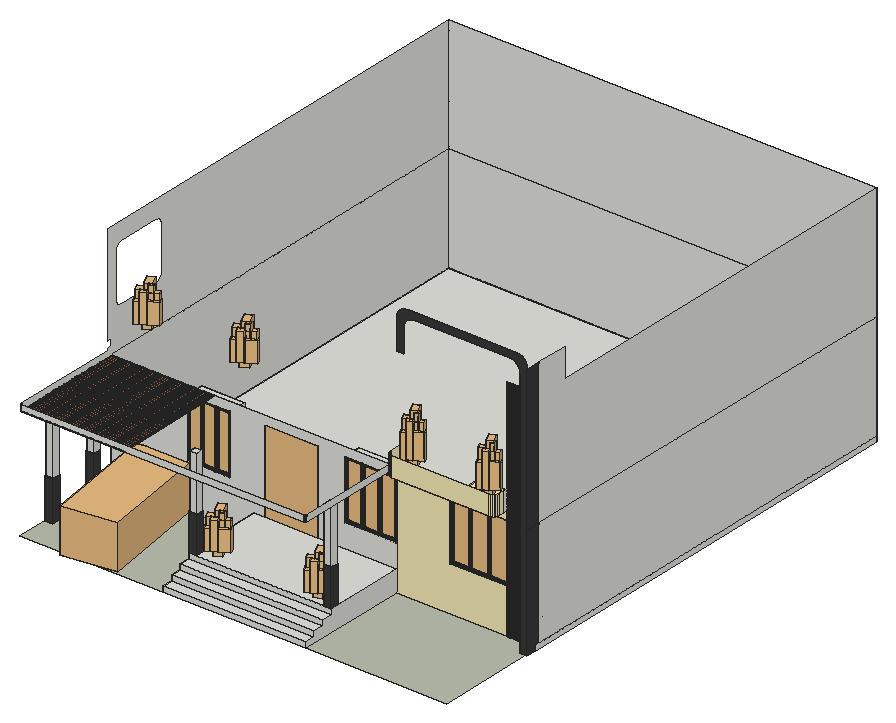
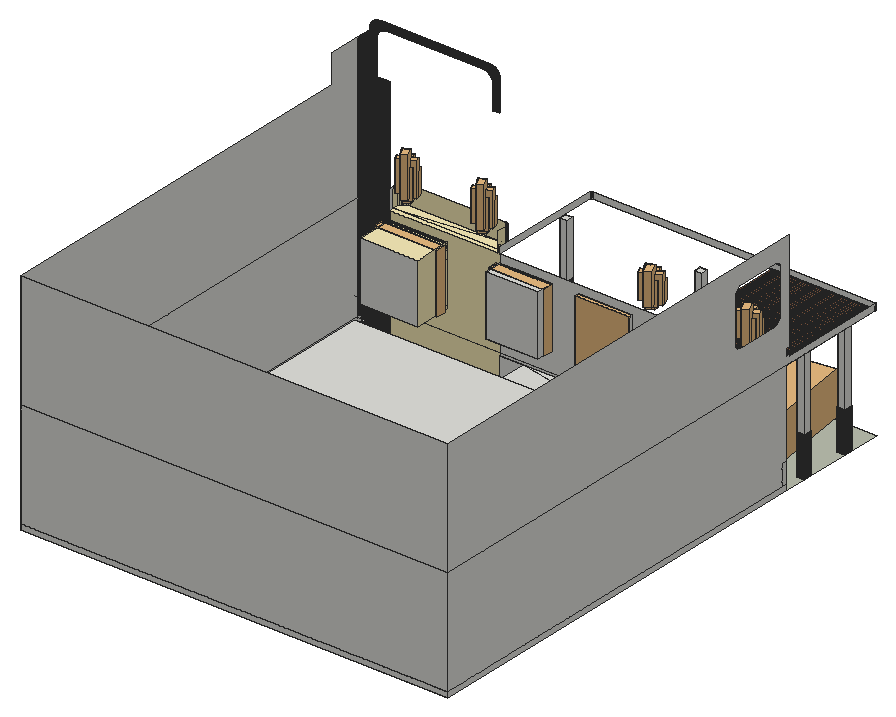
# SketchUp Ruby script. Lengths in inches.
U = 1.inch
M = Sketchup.active_model
def pt(a) = Geom::Point3d.new(a.map { |v| v * U })
def face(e, loops, mat)
  f = e.add_face(loops[0].map { |a| pt(a) })
  loops[1..].each { |l| e.add_face(l.map { |a| pt(a) }).erase! }
  f.material = f.back_material = mat if mat
  f
end
# faces: each face lists its corners as indices into pts; further lists are holes
def faces(e, pts, list, mat = nil) = list.each { |f| face(e, (f[0].is_a?(Array) ? f : [f]).map { |l| l.map { |i| pts[i] } }, mat) }
# xy, xz, yz: faces in a plane at the given z, y or x. An outline is a flat list of corners, or four numbers for a rectangle; further outlines are holes
def ring(l) = l.size == 4 ? [[l[0], l[1]], [l[2], l[1]], [l[2], l[3]], [l[0], l[3]]] : l.each_slice(2).to_a
def flat(e, list, mat, &to3) = list.each { |f| face(e, (f[0].is_a?(Array) ? f : [f]).map { |l| ring(l).map { |u, v| to3.(u, v) } }, mat) }
def xy(e, z, list, mat = nil) = flat(e, list, mat) { |x, y| [x, y, z] }
def xz(e, y, list, mat = nil) = flat(e, list, mat) { |x, z| [x, y, z] }
def yz(e, x, list, mat = nil) = flat(e, list, mat) { |y, z| [x, y, z] }
def lines(e, pts, list) = list.each { |a, b| e.add_line(pt(pts[a]), pt(pts[b])) }
# prism: a flat outline (further loops are holes) pulled along v
def prism(e, loops, v, mat = nil)
  f = face(e, loops, mat); d = Geom::Vector3d.new(v.map { |x| x * U })
  f.pushpull(f.normal.samedirection?(d) ? d.length : -d.length)
end
def box(e, o, s, mat = nil) = prism(e, [[o, [o[0] + s[0], o[1], o[2]], [o[0] + s[0], o[1] + s[1], o[2]], [o[0], o[1] + s[1], o[2]]]], [0, 0, s[2]], mat)
def at(x, y, z, deg = 0) = Geom::Transformation.translation(pt([x, y, z])) * Geom::Transformation.rotation(ORIGIN, Z_AXIS, deg.degrees)
def axes(o, x, y, z) = Geom::Transformation.new([*x, 0, *y, 0, *z, 0, *pt(o).to_a, 1])
def part(name) = M.definitions.add(name)
# library, detail: a bought-in or finely detailed component or shape, given as its bounding box
def library(name, o, s) = part(name).tap { |d| box(d.entities, o, s) }
def detail(e, o, s) = box(e.add_group.entities, o, s)
def put(e, d, t, mat = nil) = e.add_instance(d, t).tap { |i| i.material = mat if mat }
def group(e, t, mat = nil) = e.add_group.tap { |g| g.transformation = t; g.material = mat if mat }.entities
root = M.entities
M.materials.add("0899 AP 7833 SUNKISSED").color = [249, 236, 185]
M.materials.add("POT_TEXTURE_1").color = [172, 172, 172]
M.materials.add("Wine2").color = [0, 0, 0]
M.materials["Wine2"].alpha = 0
M.materials.add("[0130_Gainsboro]").color = [39, 45, 50]
M.materials.add("[Color M07]").color = [58, 58, 58]
M.materials.add("[Pavers with Grass Brick]").color = [187, 192, 176]
M.materials.add("[Wood Veneer 02]").color = [190, 128, 91]
M.materials.add("soil1").color = [68, 55, 47]
c1 = part("Group381\#1")
prism(c1.entities,[[[-13,124.5,0],[-13,-124.5,0],[-14,-124.5,0],[-14,-80.5625,0],[-14,-13.875,0],[-14,-4.5,0],[-14,19.5,0],[-14,43.5,0],[-14,106.48,0],[-14,107.5,0],[-14,122.5625,0],[-14,124.5,0]]],[0,0,0.25])
c2 = part("Group382\#1")
box(c2.entities,[-12.6875,-124.5,0],[1,249,0.25])
c3 = part("Group383\#1")
box(c3.entities,[-11.375,-124.5,0],[1,249,0.25])
c4 = part("Group384\#1")
box(c4.entities,[-10.0625,-124.5,0],[1,249,0.25])
c5 = part("Group385\#1")
box(c5.entities,[-8.75,-124.5,0],[1,249,0.25])
c6 = part("Group386\#1")
box(c6.entities,[-7.4375,-124.5,0],[1,249,0.25])
c7 = part("Group387\#1")
box(c7.entities,[-6.125,-124.5,0],[1,249,0.25])
c8 = part("Group388\#1")
box(c8.entities,[-4.8125,-124.5,0],[1,249,0.25])
c9 = part("Group389\#1")
box(c9.entities,[-3.5,-124.5,0],[1,249,0.25])
c10 = part("Group390\#1")
box(c10.entities,[-2.1875,-124.5,0],[1,249,0.25])
c11 = part("Group391\#1")
box(c11.entities,[-0.875,-124.5,0],[1,249,0.25])
c12 = part("Group392\#1")
box(c12.entities,[0.4375,-124.5,0],[1,249,0.25])
c13 = part("Group393\#1")
box(c13.entities,[1.75,-124.5,0],[1,249,0.25])
c14 = part("Group394\#1")
box(c14.entities,[3.0625,-124.5,0],[1,249,0.25])
c15 = part("Group395\#1")
box(c15.entities,[4.375,-124.5,0],[1,249,0.25])
c16 = part("Group396\#1")
box(c16.entities,[5.6875,-124.5,0],[1,249,0.25])
c17 = part("Group397\#1")
box(c17.entities,[7,-124.5,0],[1,249,0.25])
c18 = part("Group398\#1")
box(c18.entities,[8.3125,-124.5,0],[1,249,0.25])
c19 = part("Group399\#1")
box(c19.entities,[9.625,-124.5,0],[1,249,0.25])
c20 = part("Group400\#1")
box(c20.entities,[10.9375,-124.5,0],[1,249,0.25])
c21 = part("Group401\#1")
box(c21.entities,[12.25,-124.5,0],[1,249,0.25])
c22 = part("Group402\#1")
xy(c22.entities,0,[[13.5625,-124.5,14,124.5]])
xy(c22.entities,0.25,[[13.5625,-124.5,14,124.5]])
yz(c22.entities,13.5625,[[-124.5,0,124.5,0.25]])
c23 = part("Group379\#2")
put(c23.entities,c1,at(0,0,0))
put(c23.entities,c2,at(0,0,0))
put(c23.entities,c3,at(0,0,0))
put(c23.entities,c4,at(0,0,0))
put(c23.entities,c5,at(0,0,0))
put(c23.entities,c6,at(0,0,0))
put(c23.entities,c7,at(0,0,0))
put(c23.entities,c8,at(0,0,0))
put(c23.entities,c9,at(0,0,0))
put(c23.entities,c10,at(0,0,0))
put(c23.entities,c11,at(0,0,0))
put(c23.entities,c12,at(0,0,0))
put(c23.entities,c13,at(0,0,0))
put(c23.entities,c14,at(0,0,0))
put(c23.entities,c15,at(0,0,0))
put(c23.entities,c16,at(0,0,0))
put(c23.entities,c17,at(0,0,0))
put(c23.entities,c18,at(0,0,0))
put(c23.entities,c19,at(0,0,0))
put(c23.entities,c20,at(0,0,0))
put(c23.entities,c21,at(0,0,0))
put(c23.entities,c22,at(0,0,0))
c24 = library("Lexus+LX570+2016",[13.08,-4.5,0.2],[90.19,198.97,73.68])
c25 = library("Group\#94",[-662.41,217.3,320.04],[397.32,658.3,1732.06])
c26 = library("Group\#96",[-299.2,181.55,262.58],[360.65,735.71,1258.34])
c27 = library("Group\#91",[-1038.76,656.55,345.34],[733.18,460.51,2065.7])
c28 = library("Group\#89",[-445.29,890.31,329.28],[284.3,304.08,2023.29])
c29 = library("Group\#92",[-733.48,439.625,202.64],[456.28,533.12,1536.78])
c30 = library("Group\#95",[-455.56,899.32,410.78],[341.21,610.33,1581.5])
c31 = library("Group\#88",[-516.34,626.77,-4.5625],[517.73,515.95,418.98])
c32 = library("Group\#93",[-249.24,914.85,310.18],[345.55,647.95,1307.93])
c33 = library("Group\#90",[-277.97,488.68,287.26],[362.84,405.94,1768.54])
c34 = library("Group\#87",[-468.76,669.89,380.1875],[424.36,427.47,41.99])
c35 = part("Potted plant")
put(c35.entities,c25,at(1038.76,-181.55,4.5625))
put(c35.entities,c26,at(1038.76,-181.55,4.5625))
put(c35.entities,c27,at(1038.76,-181.55,4.5625))
put(c35.entities,c28,at(1038.76,-181.55,4.5625))
put(c35.entities,c29,at(1038.76,-181.55,4.5625))
put(c35.entities,c30,at(1038.76,-181.55,4.5625))
put(c35.entities,c31,at(1038.76,-181.55,4.5625),"POT_TEXTURE_1")
put(c35.entities,c32,at(1038.76,-181.55,4.5625))
put(c35.entities,c33,at(1038.76,-181.55,4.5625))
put(c35.entities,c34,at(1038.76,-181.55,4.5625),"soil1")
c36 = part("plants(2)")
put(c36.entities,c35,axes([-3298.7,16879.33,962.02],[0.26233,-0.53859,0],[0.53859,0.26233,0],[0,0,0.59908]))
put(c36.entities,c35,axes([-7168.4,16988.26,962.02],[0.26361,-0.54122,0],[0.54122,0.26361,0],[0,0,0.602]))
put(c36.entities,c35,axes([-1678.07,19377.75,4834.08],[0.22822,-0.46857,0],[0.47934,0.23347,0],[0,0,0.74285]))
put(c36.entities,c35,axes([1189.32,19377.75,4834.08],[0.22822,-0.46857,0],[0.47934,0.23347,0],[0,0,0.74285]))
put(c36.entities,c35,axes([-8907.24,20412.17,5238.12],[0.26361,-0.54122,0],[0.54122,0.26361,0],[0,0,0.602]))
put(c36.entities,c35,axes([-12589.9,20412.17,5238.12],[0.26361,-0.54122,0],[0.54122,0.26361,0],[0,0,0.602]))
c37 = library("Double Door",[0,-0.98,0],[62,4.92,84])
c38 = library("шторы раздвинутые\#1",[23.6875,-79.37,-3.6],[68.3125,79.85,10.87])
c39 = part("Window sash")
xy(c39.entities,0,[[0,-0.98,43.07,0],[0,0,43.07,1.4]],"[0130_Gainsboro]")
xy(c39.entities,0.3,[[0.3,-1.43,42.77,-0.98]],"[0130_Gainsboro]")
xy(c39.entities,2.95,[[2.95,-1.43,40.12,-0.63],[2.95,-0.63,40.12,0],[2.95,0,40.12,0.64],[2.95,0.64,40.12,1.4]],"[0130_Gainsboro]")
xy(c39.entities,3.54,[[3.54,-0.63,39.53,0],[3.54,0,39.53,0.64]],"[0130_Gainsboro]")
xy(c39.entities,111.8125,[[3.54,-0.63,39.53,0],[3.54,0,39.53,0.64]],"[0130_Gainsboro]")
xy(c39.entities,112.4,[[2.95,-1.43,40.12,-0.63],[2.95,-0.63,40.12,0],[2.95,0,40.12,0.64],[2.95,0.64,40.12,1.4]],"[0130_Gainsboro]")
xy(c39.entities,115.05,[[0.3,-1.43,42.77,-0.98]],"[0130_Gainsboro]")
xy(c39.entities,115.35,[[0,-0.98,43.07,0],[0,0,43.07,1.4]],"[0130_Gainsboro]")
xz(c39.entities,-1.43,[[[0.3,0.3,42.77,115.05],[2.95,2.95,40.12,112.4]]],"[0130_Gainsboro]")
xz(c39.entities,-0.98,[[[0,0,43.07,115.35],[0.3,0.3,42.77,115.05]]],"[0130_Gainsboro]")
xz(c39.entities,-0.63,[[[2.95,2.95,40.12,112.4],[3.54,3.54,39.53,111.8125]]],"[0130_Gainsboro]")
xz(c39.entities,0,[[3.54,3.54,39.53,111.8125]],"Wine2")
xz(c39.entities,0,[[[0,0,43.07,115.35],[2.95,2.95,40.12,112.4]],[[2.95,2.95,40.12,112.4],[3.54,3.54,39.53,111.8125]]],"[0130_Gainsboro]")
xz(c39.entities,0.64,[[[2.95,2.95,40.12,112.4],[3.54,3.54,39.53,111.8125]]],"[0130_Gainsboro]")
xz(c39.entities,1.4,[[[0,0,43.07,115.35],[2.95,2.95,40.12,112.4]]],"[0130_Gainsboro]")
yz(c39.entities,0,[[-0.98,0,0,115.35],[0,0,1.4,115.35]],"[0130_Gainsboro]")
yz(c39.entities,0.3,[[-1.43,0.3,-0.98,115.05]],"[0130_Gainsboro]")
yz(c39.entities,2.95,[[-1.43,2.95,-0.63,112.4],[-0.63,2.95,0,112.4],[0,2.95,0.64,112.4],[0.64,2.95,1.4,112.4]],"[0130_Gainsboro]")
yz(c39.entities,3.54,[[-0.63,3.54,0,111.8125],[0,3.54,0.64,111.8125]],"[0130_Gainsboro]")
yz(c39.entities,39.53,[[-0.63,3.54,0,111.8125],[0,3.54,0.64,111.8125]],"[0130_Gainsboro]")
yz(c39.entities,40.12,[[-1.43,2.95,-0.63,112.4],[-0.63,2.95,0,112.4],[0,2.95,0.64,112.4],[0.64,2.95,1.4,112.4]],"[0130_Gainsboro]")
yz(c39.entities,42.77,[[-1.43,0.3,-0.98,115.05]],"[0130_Gainsboro]")
yz(c39.entities,43.07,[[-0.98,0,0,115.35],[0,0,1.4,115.35]],"[0130_Gainsboro]")
c40 = part("Three-panel window")
put(c40.entities,c39,axes([90.57,1.43,0],[1.05148,0,0],[0,1,0],[0,0,1]))
put(c40.entities,c39,axes([0,1.43,0],[1.05148,0,0],[0,1,0],[0,0,1]))
put(c40.entities,c39,axes([45.29,1.43,0],[1.05148,0,0],[0,1,0],[0,0,1]))
c41 = part("Group614\#1")
xy(c41.entities,0,[[-159,-63.39,-159.09,-63.37,-159.49,-63.08,-159.77,-62.68,-159.94,-62.16,-160,-61.54,-160,63.59,-159,63.59]])
xy(c41.entities,0.24,[[-159,-63.39,-159,63.59,-160,63.59,-160,-61.54,-159.94,-62.16,-159.77,-62.68,-159.49,-63.08,-159.09,-63.37]])
yz(c41.entities,-160,[[-61.54,0,63.59,0.24]])
yz(c41.entities,-159,[[-63.39,0,63.59,0.24]])
c42 = part("Group615\#1")
xy(c42.entities,0,[[-157.94,-63.59,-158.57,-63.54,-158.7,-63.49,-158.7,63.59,-157.7,63.59,-157.7,-63.59]])
xy(c42.entities,0.24,[[-157.94,-63.59,-157.7,-63.59,-157.7,63.59,-158.7,63.59,-158.7,-63.49,-158.57,-63.54]])
xz(c42.entities,63.59,[[-158.7,0,-157.7,0.24]])
yz(c42.entities,-158.7,[[-63.49,0,63.59,0.24]])
yz(c42.entities,-157.7,[[-63.59,0,63.59,0.24]])
c43 = part("Group616\#1")
box(c43.entities,[-157.4,-63.59,0],[1,127.18,0.24])
c44 = part("Group617\#1")
box(c44.entities,[-156.1,-63.59,0],[1,127.18,0.24])
c45 = part("Group618\#1")
box(c45.entities,[-154.8,-63.59,0],[1,127.18,0.24])
c46 = part("Group619\#1")
box(c46.entities,[-153.5,-63.59,0],[1,127.18,0.24])
c47 = part("Group620\#1")
box(c47.entities,[-152.2,-63.59,0],[1,127.18,0.24])
c48 = part("Group621\#1")
box(c48.entities,[-150.9,-63.59,0],[1,127.18,0.24])
c49 = part("Group622\#1")
box(c49.entities,[-149.6,-63.59,0],[1,127.18,0.24])
c50 = part("Group623\#1")
box(c50.entities,[-148.3,-63.59,0],[1,127.18,0.24])
c51 = part("Group624\#1")
box(c51.entities,[-147,-63.59,0],[1,127.18,0.24])
c52 = part("Group625\#1")
box(c52.entities,[-145.7,-63.59,0],[1,127.18,0.24])
c53 = part("Group626\#1")
box(c53.entities,[-144.4,-63.59,0],[1,127.18,0.24])
c54 = part("Group627\#1")
box(c54.entities,[-143.1,-63.59,0],[1,127.18,0.24])
c55 = part("Group628\#1")
box(c55.entities,[-141.8,-63.59,0],[1,127.18,0.24])
c56 = part("Group629\#1")
box(c56.entities,[-140.5,-63.59,0],[1,127.18,0.24])
c57 = part("Group630\#1")
box(c57.entities,[-139.2,-63.59,0],[1,127.18,0.24])
c58 = part("Group631\#1")
box(c58.entities,[-137.9,-63.59,0],[1,127.18,0.24])
c59 = part("Group632\#1")
box(c59.entities,[-136.6,-63.59,0],[1,127.18,0.24])
c60 = part("Group633\#1")
box(c60.entities,[-135.3,-63.59,0],[1,127.18,0.24])
c61 = part("Group634\#1")
box(c61.entities,[-134,-63.59,0],[1,127.18,0.24])
c62 = part("Group635\#1")
box(c62.entities,[-132.7,-63.59,0],[1,127.18,0.24])
c63 = part("Group636\#1")
box(c63.entities,[-131.4,-63.59,0],[1,127.18,0.24])
c64 = part("Group637\#1")
box(c64.entities,[-130.1,-63.59,0],[1,127.18,0.24])
c65 = part("Group638\#1")
box(c65.entities,[-128.8,-63.59,0],[1,127.18,0.24])
c66 = part("Group639\#1")
box(c66.entities,[-127.5,-63.59,0],[1,127.18,0.24])
c67 = part("Group640\#1")
box(c67.entities,[-126.2,-63.59,0],[1,127.18,0.24])
c68 = part("Group641\#1")
box(c68.entities,[-124.9,-63.59,0],[1,127.18,0.24])
c69 = part("Group642\#1")
box(c69.entities,[-123.6,-63.59,0],[1,127.18,0.24])
c70 = part("Group643\#1")
box(c70.entities,[-122.3,-63.59,0],[1,127.18,0.24])
c71 = part("Group644\#1")
box(c71.entities,[-121,-63.59,0],[1,127.18,0.24])
c72 = part("Group645\#1")
box(c72.entities,[-119.7,-63.59,0],[1,127.18,0.24])
c73 = part("Group646\#1")
box(c73.entities,[-118.4,-63.59,0],[1,127.18,0.24])
c74 = part("Group647\#1")
box(c74.entities,[-117.1,-63.59,0],[1,127.18,0.24])
c75 = part("Group648\#1")
box(c75.entities,[-115.8,-63.59,0],[1,127.18,0.24])
c76 = part("Group649\#1")
box(c76.entities,[-114.5,-63.59,0],[1,127.18,0.24])
c77 = part("Group650\#1")
box(c77.entities,[-113.2,-63.59,0],[1,127.18,0.24])
c78 = part("Group651\#1")
box(c78.entities,[-111.9,-63.59,0],[1,127.18,0.24])
c79 = part("Group652\#1")
box(c79.entities,[-110.6,-63.59,0],[1,127.18,0.24])
c80 = part("Group653\#1")
box(c80.entities,[-109.3,-63.59,0],[1,127.18,0.24])
c81 = part("Group654\#1")
box(c81.entities,[-108,-63.59,0],[1,127.18,0.24])
c82 = part("Group655\#1")
box(c82.entities,[-106.7,-63.59,0],[1,127.18,0.24])
c83 = part("Group656\#1")
box(c83.entities,[-105.4,-63.59,0],[1,127.18,0.24])
c84 = part("Group657\#1")
box(c84.entities,[-104.1,-63.59,0],[1,127.18,0.24])
c85 = part("Group658\#1")
box(c85.entities,[-102.8,-63.59,0],[1,127.18,0.24])
c86 = part("Group659\#1")
box(c86.entities,[-101.5,-63.59,0],[1,127.18,0.24])
c87 = part("Group660\#1")
box(c87.entities,[-100.2,-63.59,0],[1,127.18,0.24])
c88 = part("Group661\#1")
box(c88.entities,[-98.9,-63.59,0],[1,127.18,0.24])
c89 = part("Group662\#1")
box(c89.entities,[-97.6,-63.59,0],[1,127.18,0.24])
c90 = part("Group663\#1")
box(c90.entities,[-96.3,-63.59,0],[1,127.18,0.24])
c91 = part("Group664\#1")
box(c91.entities,[-95,-63.59,0],[1,127.18,0.24])
c92 = part("Group665\#1")
box(c92.entities,[-93.7,-63.59,0],[1,127.18,0.24])
c93 = part("Group666\#1")
box(c93.entities,[-92.4,-63.59,0],[1,127.18,0.24])
c94 = part("Group667\#1")
box(c94.entities,[-91.1,-63.59,0],[1,127.18,0.24])
c95 = part("Group668\#1")
box(c95.entities,[-89.8,-63.59,0],[1,127.18,0.24])
c96 = part("Group669\#1")
box(c96.entities,[-88.5,-63.59,0],[1,127.18,0.24])
c97 = part("Group670\#1")
box(c97.entities,[-87.2,-63.59,0],[1,127.18,0.24])
c98 = part("Group671\#1")
box(c98.entities,[-85.9,-63.59,0],[1,127.18,0.24])
c99 = part("Group672\#1")
box(c99.entities,[-84.6,-63.59,0],[1,127.18,0.24])
c100 = part("Group673\#1")
box(c100.entities,[-83.3,-63.59,0],[1,127.18,0.24])
c101 = part("Group674\#1")
box(c101.entities,[-82,-63.59,0],[1,127.18,0.24])
c102 = part("Group675\#1")
box(c102.entities,[-80.7,-63.59,0],[1,127.18,0.24])
c103 = part("Group676\#1")
box(c103.entities,[-79.4,-63.59,0],[1,127.18,0.24])
c104 = part("Group677\#1")
box(c104.entities,[-78.1,-63.59,0],[1,127.18,0.24])
c105 = part("Group678\#1")
box(c105.entities,[-76.8,-63.59,0],[1,127.18,0.24])
c106 = part("Group679\#1")
box(c106.entities,[-75.5,-63.59,0],[1,127.18,0.24])
c107 = part("Group680\#1")
box(c107.entities,[-74.2,-63.59,0],[1,127.18,0.24])
c108 = part("Group681\#1")
box(c108.entities,[-72.9,-63.59,0],[1,127.18,0.24])
c109 = part("Group682\#1")
box(c109.entities,[-71.6,-63.59,0],[1,127.18,0.24])
c110 = part("Group683\#1")
box(c110.entities,[-70.3,-63.59,0],[1,127.18,0.24])
c111 = part("Group684\#1")
box(c111.entities,[-69,-63.59,0],[1,127.18,0.24])
c112 = part("Group685\#1")
box(c112.entities,[-67.7,-63.59,0],[1,127.18,0.24])
c113 = part("Group686\#1")
box(c113.entities,[-66.4,-63.59,0],[1,127.18,0.24])
c114 = part("Group687\#1")
box(c114.entities,[-65.1,-63.59,0],[1,127.18,0.24])
c115 = part("Group688\#1")
box(c115.entities,[-63.8,-63.59,0],[1,127.18,0.24])
c116 = part("Group689\#1")
box(c116.entities,[-62.5,-63.59,0],[1,127.18,0.24])
c117 = part("Group690\#1")
box(c117.entities,[-61.2,-63.59,0],[1,127.18,0.24])
c118 = part("Group691\#1")
box(c118.entities,[-59.9,-63.59,0],[1,127.18,0.24])
c119 = part("Group692\#1")
box(c119.entities,[-58.6,-63.59,0],[1,127.18,0.24])
c120 = part("Group693\#1")
box(c120.entities,[-57.3,-63.59,0],[1,127.18,0.24])
c121 = part("Group694\#1")
box(c121.entities,[-56,-63.59,0],[1,127.18,0.24])
c122 = part("Group695\#1")
box(c122.entities,[-54.7,-63.59,0],[1,127.18,0.24])
c123 = part("Group696\#1")
box(c123.entities,[-53.4,-63.59,0],[1,127.18,0.24])
c124 = part("Group697\#1")
box(c124.entities,[-52.1,-63.59,0],[1,127.18,0.24])
c125 = part("Group698\#1")
box(c125.entities,[-50.8,-63.59,0],[1,127.18,0.24])
c126 = part("Group699\#1")
box(c126.entities,[-49.5,-63.59,0],[1,127.18,0.24])
c127 = part("Group700\#1")
box(c127.entities,[-48.2,-63.59,0],[1,127.18,0.24])
c128 = part("Group701\#1")
box(c128.entities,[-46.9,-63.59,0],[1,127.18,0.24])
c129 = part("Group702\#1")
box(c129.entities,[-45.6,-63.59,0],[1,127.18,0.24])
c130 = part("Group703\#1")
box(c130.entities,[-44.3,-63.59,0],[1,127.18,0.24])
xy(root,0,[[161,1,321,128.1875],[473,111.1875,473,128.1875,479.375,123.1875,479.375,111.1875],[479.375,111.1875,481,123.1875],[479.375,123.1875,473,128.1875,1,128.1875,1,601,481,601,481,123.1875]])
xy(root,0,[[1,1,161,128.1875],[321,1,479.375,1,479.375,111.1875,473,111.1875,473,128.1875,321,128.1875]],"[Pavers with Grass Brick]")
xy(root,6,[[161,1,321,13],[1,133,481,601]])
xy(root,12,[[161,13,321,25]])
xy(root,18,[[161,25,321,37]])
xy(root,24,[[161,37,313,37,313,45,321,45,321,128.1875,233,128.1875,233,131.8125,173,131.8125,173,128.1875,161,128.1875]])
xy(root,49.9375,[[86.625,128.1875,134.625,148.3125],[263,128.1875,321,148.3125]])
xy(root,49.9375,[[380.875,128.1875,445,169.5625]],"0899 AP 7833 SUNKISSED")
xy(root,116.625,[[86.625,128.1875,134.625,148.3125],[173,128.1875,233,131.8125],[263,128.1875,321,148.3125]])
xy(root,116.625,[[380.875,128.1875,445,169.5625]],"0899 AP 7833 SUNKISSED")
xy(root,126,[[330.04,111.1875,328.1,111.36,326.51,111.89,325.28,112.78,324.39,114.01,323.86,115.6,323.6875,117.54,323.6875,123.1875,445,123.1875,445,117.54,444.82,115.6,444.29,114.01,443.41,112.78,442.18,111.89,440.59,111.36,438.65,111.1875],[323.6875,123.1875,445,128.1875]],"0899 AP 7833 SUNKISSED")
xz(root,1,[[161,0,321,6],[3.06,126,318.94,133]])
xz(root,13,[[161,6,321,12]])
xz(root,25,[[161,12,321,18]])
xz(root,37,[[161,18,321,24]])
xz(root,111.1875,[[330.04,126,438.65,148]],"0899 AP 7833 SUNKISSED")
xz(root,111.1875,[[473,0,481,0,481,287.51,480.625,291.63,479.5,295.01,477.63,297.63,475.01,299.5,471.63,300.625,467.51,301,348.2,301,344.08,300.625,340.71,299.5,338.08,297.63,336.21,295.01,335.09,291.63,334.71,287.51,334.71,255,342.71,255,342.71,279.51,343.09,283.63,344.21,287.01,346.08,289.63,348.71,291.5,352.08,292.625,356.2,293,459.51,293,463.63,292.625,467.01,291.5,469.63,289.63,471.5,287.01,472.625,283.63,473,279.51]],"[Color M07]")
xz(root,128.1875,[[[1,0,161,0,161,24,173,24,173,116.625,233,116.625,233,24,321,24,321,0,322,0,322,133,321,133,321,126,1,126],[263,49.9375,321,116.625],[86.625,49.9375,134.625,116.625]],[445,0,473,6]])
xz(root,128.1875,[[322,0,445,0,445,49.9375,380.875,49.9375,380.875,116.625,445,116.625,445,126,323.6875,126,323.6875,135,322,135]],"0899 AP 7833 SUNKISSED")
xz(root,131.8125,[[173,24,233,116.625]])
xz(root,148.3125,[[86.625,49.9375,134.625,116.625],[263,49.9375,321,116.625]])
xz(root,169.5625,[[380.875,49.9375,445,116.625]])
xz(root,601,[[1,0,481,6],[1,6,481,126],[1,126,481,255]])
yz(root,1,[[128.1875,0,601,6],[128.1875,6,133,30],[133,6,133,30,128.1875,30,128.1875,126,601,126,601,6],[[3.06,126,3.06,133,123.1875,133,123.1875,135,128.1875,135,128.1875,143,123.1875,143,123.1875,255,601,255,601,126],[143.3,171,191.01,171,193.49,171.23,195.52,171.9,197.1,173.03,198.22,174.61,198.9,176.63,199.125,179.11,199.125,226.89,198.9,229.37,198.22,231.39,197.1,232.97,195.52,234.1,193.49,234.77,191.01,235,143.3,235,140.82,234.77,138.79,234.1,137.22,232.97,136.09,231.39,135.41,229.37,135.1875,226.89,135.1875,179.11,135.41,176.63,136.09,174.61,137.22,173.03,138.79,171.9,140.82,171.23]]])
yz(root,86.625,[[128.1875,49.9375,148.3125,116.625]])
yz(root,134.625,[[128.1875,49.9375,148.3125,116.625]])
yz(root,161,[[1,0,1,6,13,6,13,12,25,12,25,18,37,18,37,24,128.1875,24,128.1875,0]])
yz(root,173,[[128.1875,24,131.8125,116.625]])
yz(root,233,[[128.1875,24,131.8125,116.625]])
yz(root,263,[[128.1875,49.9375,148.3125,116.625]])
yz(root,321,[[1,0,128.1875,0,128.1875,24,37,24,37,18,25,18,25,12,13,12,13,6,1,6],[128.1875,49.9375,148.3125,116.625],[3.06,126,128.1875,133]])
yz(root,323.6875,[[117.54,126,128.1875,148]],"0899 AP 7833 SUNKISSED")
yz(root,380.875,[[128.1875,49.9375,169.5625,116.625]],"0899 AP 7833 SUNKISSED")
yz(root,445,[[123.1875,126,128.1875,148.01]])
yz(root,445,[[128.1875,49.9375,169.5625,116.625],[117.54,126,123.1875,148]],"0899 AP 7833 SUNKISSED")
yz(root,473,[[111.1875,0,128.1875,279.51]],"[Color M07]")
yz(root,481,[[123.1875,0,601,6],[128.1875,6,601,126],[128.1875,126,601,126,601,255,164.1875,255,164.1875,287.51,128.1875,287.51]])
yz(root,481,[[111.1875,0,123.1875,0,123.1875,6,128.1875,6,128.1875,126,111.1875,126],[111.1875,126,128.1875,287.51]],"[Color M07]")
p = [[3.06,1,126],[3.06,1,133],[2.43,1.06,133],[2.43,1.06,126],[318.94,1,133],[318.94,1,126],
  [319.57,1.06,126],[319.57,1.06,133],[1.91,1.23,133],[1.91,1.23,126],[320.09,1.23,126],[320.09,1.23,133],
  [1.51,1.51,133],[1.51,1.51,126],[320.49,1.51,126],[320.49,1.51,133],[1.23,1.91,133],[1.23,1.91,126],
  [320.77,1.91,126],[320.77,1.91,133],[1.06,2.43,133],[1.06,2.43,126],[320.94,2.43,126],[320.94,2.43,133],
  [1,3.06,133],[1,3.06,126],[321,3.06,126],[321,3.06,133],[330.04,111.1875,126],[330.04,111.1875,148],
  [328.1,111.36,148],[328.1,111.36,126],[440.59,111.36,126],[440.59,111.36,148],[438.65,111.1875,148],[438.65,111.1875,126],
  [326.51,111.89,148],[326.51,111.89,126],[442.18,111.89,126],[442.18,111.89,148],[325.28,112.78,148],[325.28,112.78,126],
  [443.41,112.78,126],[443.41,112.78,148],[324.39,114.01,148],[324.39,114.01,126],[444.29,114.01,126],[444.29,114.01,148],
  [323.92,115.4375,148],[323.86,115.6,148],[323.86,115.6,126],[444.82,115.6,126],[444.82,115.6,148],[444.77,115.4375,148],
  [323.6875,117.54,148],[323.6875,117.54,126],[445,117.54,126],[445,117.54,148],[481,133,30],[1,133,30],
  [323.6875,123.1875,135],[445,123.1875,126],[473,128.1875,6],[481,128.1875,6],[473,123.1875,6],[481,123.1875,6],
  [321,123.1875,24],[161,128.1875,0]]
faces(root,p,[[0,1,2,3],[4,5,6,7],[3,2,8,9],[7,6,10,11],[9,8,12,13],[11,10,14,15],[13,12,16,17],[15,14,18,19],
  [17,16,20,21],[19,18,22,23],[21,20,24,25],[23,22,26,27]])
faces(root,p,[[28,29,30,31],[32,33,34,35],[31,30,36,37],[38,39,33,32],[37,36,40,41],[42,43,39,38],[41,40,44,45],[46,47,43,42],
  [45,44,48,49,50],[51,52,53,47,46],[50,49,54,55],[56,57,52,51]],"0899 AP 7833 SUNKISSED")
lines(root,p,[[58,59],[60,61],[62,63],[64,65],[66,67]])
g1 = group(root,at(1,37,24))
xy(g1,-24,[[-0.47,-0.47,8.47,8.47]])
xy(g1,21.375,[[0,0,8,8]])
xy(g1,21.375,[[-0.47,-0.47,0,8.47],[0,-0.47,8.47,0],[8,0,8.47,8],[0,8,8.47,8.47]],"[Color M07]")
xy(g1,102,[[0,0,8,8]])
xz(g1,-0.47,[[-0.47,-24,8.47,21.375]],"[Color M07]")
xz(g1,0,[[0,21.375,8,102]])
xz(g1,8,[[0,21.375,8,102]])
xz(g1,8.47,[[-0.47,-24,8.47,21.375]],"[Color M07]")
yz(g1,-0.47,[[-0.47,-24,8.47,21.375]],"[Color M07]")
yz(g1,0,[[0,21.375,8,102]])
yz(g1,8,[[0,21.375,8,102]])
yz(g1,8.47,[[-0.47,-24,8.47,21.375]],"[Color M07]")
g2 = group(root,at(1,93.75,24))
xy(g2,-24,[[-0.47,-0.47,8.47,8.47]])
xy(g2,21.375,[[0,0,8,8]])
xy(g2,21.375,[[-0.47,-0.47,0,8.47],[0,-0.47,8.47,0],[8,0,8.47,8],[0,8,8.47,8.47]],"[Color M07]")
xy(g2,102,[[0,0,8,8]])
xz(g2,-0.47,[[-0.47,-24,8.47,21.375]],"[Color M07]")
xz(g2,0,[[0,21.375,8,102]])
xz(g2,8,[[0,21.375,8,102]])
xz(g2,8.47,[[-0.47,-24,8.47,21.375]],"[Color M07]")
yz(g2,-0.47,[[-0.47,-24,8.47,21.375]],"[Color M07]")
yz(g2,0,[[0,21.375,8,102]])
yz(g2,8,[[0,21.375,8,102]])
yz(g2,8.47,[[-0.47,-24,8.47,21.375]],"[Color M07]")
put(root,c23,axes([459,128.1875,127.5],[1,0,0],[0,0,1.0241],[0,-1,0]),"[Wood Veneer 02]")
put(root,c24,axes([39.63,-1.66,0.07],[0.65309,0.09528,0],[-0.09528,0.65309,0],[0,0,0.66]))
put(root,c36,axes([378.49,-445.58,-4.57],[0.0297,0,0],[0,0.0297,0],[0,0,0.0297]))
put(root,c37,axes([173,129.17,24],[0.96774,0,0],[0,1,0],[0,0,1.10268]))
g3 = group(root,at(161.47,37.47,24))
xy(g3,0,[[-0.47,-0.47,8.47,8.47]])
xy(g3,41.41,[[0,0,8,8]])
xy(g3,41.41,[[-0.47,-0.47,8,0],[8,-0.47,8.47,8],[-0.47,0,0,8],[-0.47,8,8.47,8.47]],"[Color M07]")
xy(g3,102,[[0,0,8,8]])
xz(g3,-0.47,[[-0.47,0,8.47,41.41]],"[Color M07]")
xz(g3,0,[[0,41.41,8,102]])
xz(g3,8,[[0,41.41,8,102]])
xz(g3,8.47,[[-0.47,0,8.47,41.41]],"[Color M07]")
yz(g3,-0.47,[[-0.47,0,8.47,41.41]],"[Color M07]")
yz(g3,0,[[0,41.41,8,102]])
yz(g3,8,[[0,41.41,8,102]])
yz(g3,8.47,[[-0.47,0,8.47,41.41]],"[Color M07]")
p = [[0,8.47,41.41],[0,8.6875,41.41]]
lines(g3,p,[[0,1]])
g4 = group(root,at(312.53,37.4375,24))
xy(g4,0,[[-0.47,-0.47,8.47,8.47]])
xy(g4,41.41,[[0,0,8,8]])
xy(g4,41.41,[[-0.47,-0.47,8,0],[8,-0.47,8.47,8.47],[-0.47,0,0,8.47],[0,8,8,8.47]],"[Color M07]")
xy(g4,102,[[0,0,8,8]])
xz(g4,-0.47,[[-0.47,0,8.47,41.41]],"[Color M07]")
xz(g4,0,[[0,41.41,8,102]])
xz(g4,8,[[0,41.41,8,102]])
xz(g4,8.47,[[-0.47,0,8.47,41.41]],"[Color M07]")
yz(g4,-0.47,[[-0.47,0,8.47,41.41]],"[Color M07]")
yz(g4,0,[[0,41.41,8,102]])
yz(g4,8,[[0,41.41,8,102]])
yz(g4,8.47,[[-0.47,0,8.47,41.41]],"[Color M07]")
put(root,c38,axes([239.48,137.66,116.61],[0.9156,0,0],[0,0,0.84006],[0,-1,0]))
put(root,c40,axes([86.625,128.1875,49.9375],[0.3533,0,0],[0,1,0],[0,0,0.57811]))
put(root,c38,axes([353.57,141.83,116.23],[1.03745,0,0],[0,0,0.83522],[0,-1,0]))
put(root,c40,axes([380.875,129.89,49.9375],[0.47199,0,0],[0,0.4,0],[0,0,0.57811]))
put(root,c40,axes([263,128.1875,49.9375],[0.42691,0,0],[0,1,0],[0,0,0.57811]))
put(root,c38,axes([66.65,137.66,116.61],[0.76595,0,0],[0,0,0.84006],[0,-1,0]))
put(root,c41,at(161,64.59,126),"[Wood Veneer 02]")
put(root,c42,at(161,64.59,126),"[Wood Veneer 02]")
put(root,c43,at(161,64.59,126),"[Wood Veneer 02]")
put(root,c44,at(161,64.59,126),"[Wood Veneer 02]")
put(root,c45,at(161,64.59,126),"[Wood Veneer 02]")
put(root,c46,at(161,64.59,126),"[Wood Veneer 02]")
put(root,c47,at(161,64.59,126),"[Wood Veneer 02]")
put(root,c48,at(161,64.59,126),"[Wood Veneer 02]")
put(root,c49,at(161,64.59,126),"[Wood Veneer 02]")
put(root,c50,at(161,64.59,126),"[Wood Veneer 02]")
put(root,c51,at(161,64.59,126),"[Wood Veneer 02]")
put(root,c52,at(161,64.59,126),"[Wood Veneer 02]")
put(root,c53,at(161,64.59,126),"[Wood Veneer 02]")
put(root,c54,at(161,64.59,126),"[Wood Veneer 02]")
put(root,c55,at(161,64.59,126),"[Wood Veneer 02]")
put(root,c56,at(161,64.59,126),"[Wood Veneer 02]")
put(root,c57,at(161,64.59,126),"[Wood Veneer 02]")
put(root,c58,at(161,64.59,126),"[Wood Veneer 02]")
put(root,c59,at(161,64.59,126),"[Wood Veneer 02]")
put(root,c60,at(161,64.59,126),"[Wood Veneer 02]")
put(root,c61,at(161,64.59,126),"[Wood Veneer 02]")
put(root,c62,at(161,64.59,126),"[Wood Veneer 02]")
put(root,c63,at(161,64.59,126),"[Wood Veneer 02]")
put(root,c64,at(161,64.59,126),"[Wood Veneer 02]")
put(root,c65,at(161,64.59,126),"[Wood Veneer 02]")
put(root,c66,at(161,64.59,126),"[Wood Veneer 02]")
put(root,c67,at(161,64.59,126),"[Wood Veneer 02]")
put(root,c68,at(161,64.59,126),"[Wood Veneer 02]")
put(root,c69,at(161,64.59,126),"[Wood Veneer 02]")
put(root,c70,at(161,64.59,126),"[Wood Veneer 02]")
put(root,c71,at(161,64.59,126),"[Wood Veneer 02]")
put(root,c72,at(161,64.59,126),"[Wood Veneer 02]")
put(root,c73,at(161,64.59,126),"[Wood Veneer 02]")
put(root,c74,at(161,64.59,126),"[Wood Veneer 02]")
put(root,c75,at(161,64.59,126),"[Wood Veneer 02]")
put(root,c76,at(161,64.59,126),"[Wood Veneer 02]")
put(root,c77,at(161,64.59,126),"[Wood Veneer 02]")
put(root,c78,at(161,64.59,126),"[Wood Veneer 02]")
put(root,c79,at(161,64.59,126),"[Wood Veneer 02]")
put(root,c80,at(161,64.59,126),"[Wood Veneer 02]")
put(root,c81,at(161,64.59,126),"[Wood Veneer 02]")
put(root,c82,at(161,64.59,126),"[Wood Veneer 02]")
put(root,c83,at(161,64.59,126),"[Wood Veneer 02]")
put(root,c84,at(161,64.59,126),"[Wood Veneer 02]")
put(root,c85,at(161,64.59,126),"[Wood Veneer 02]")
put(root,c86,at(161,64.59,126),"[Wood Veneer 02]")
put(root,c87,at(161,64.59,126),"[Wood Veneer 02]")
put(root,c88,at(161,64.59,126),"[Wood Veneer 02]")
put(root,c89,at(161,64.59,126),"[Wood Veneer 02]")
put(root,c90,at(161,64.59,126),"[Wood Veneer 02]")
put(root,c91,at(161,64.59,126),"[Wood Veneer 02]")
put(root,c92,at(161,64.59,126),"[Wood Veneer 02]")
put(root,c93,at(161,64.59,126),"[Wood Veneer 02]")
put(root,c94,at(161,64.59,126),"[Wood Veneer 02]")
put(root,c95,at(161,64.59,126),"[Wood Veneer 02]")
put(root,c96,at(161,64.59,126),"[Wood Veneer 02]")
put(root,c97,at(161,64.59,126),"[Wood Veneer 02]")
put(root,c98,at(161,64.59,126),"[Wood Veneer 02]")
put(root,c99,at(161,64.59,126),"[Wood Veneer 02]")
put(root,c100,at(161,64.59,126),"[Wood Veneer 02]")
put(root,c101,at(161,64.59,126),"[Wood Veneer 02]")
put(root,c102,at(161,64.59,126),"[Wood Veneer 02]")
put(root,c103,at(161,64.59,126),"[Wood Veneer 02]")
put(root,c104,at(161,64.59,126),"[Wood Veneer 02]")
put(root,c105,at(161,64.59,126),"[Wood Veneer 02]")
put(root,c106,at(161,64.59,126),"[Wood Veneer 02]")
put(root,c107,at(161,64.59,126),"[Wood Veneer 02]")
put(root,c108,at(161,64.59,126),"[Wood Veneer 02]")
put(root,c109,at(161,64.59,126),"[Wood Veneer 02]")
put(root,c110,at(161,64.59,126),"[Wood Veneer 02]")
put(root,c111,at(161,64.59,126),"[Wood Veneer 02]")
put(root,c112,at(161,64.59,126),"[Wood Veneer 02]")
put(root,c113,at(161,64.59,126),"[Wood Veneer 02]")
put(root,c114,at(161,64.59,126),"[Wood Veneer 02]")
put(root,c115,at(161,64.59,126),"[Wood Veneer 02]")
put(root,c116,at(161,64.59,126),"[Wood Veneer 02]")
put(root,c117,at(161,64.59,126),"[Wood Veneer 02]")
put(root,c118,at(161,64.59,126),"[Wood Veneer 02]")
put(root,c119,at(161,64.59,126),"[Wood Veneer 02]")
put(root,c120,at(161,64.59,126),"[Wood Veneer 02]")
put(root,c121,at(161,64.59,126),"[Wood Veneer 02]")
put(root,c122,at(161,64.59,126),"[Wood Veneer 02]")
put(root,c123,at(161,64.59,126),"[Wood Veneer 02]")
put(root,c124,at(161,64.59,126),"[Wood Veneer 02]")
put(root,c125,at(161,64.59,126),"[Wood Veneer 02]")
put(root,c126,at(161,64.59,126),"[Wood Veneer 02]")
put(root,c127,at(161,64.59,126),"[Wood Veneer 02]")
put(root,c128,at(161,64.59,126),"[Wood Veneer 02]")
put(root,c129,at(161,64.59,126),"[Wood Veneer 02]")
put(root,c130,at(161,64.59,126),"[Wood Veneer 02]")
